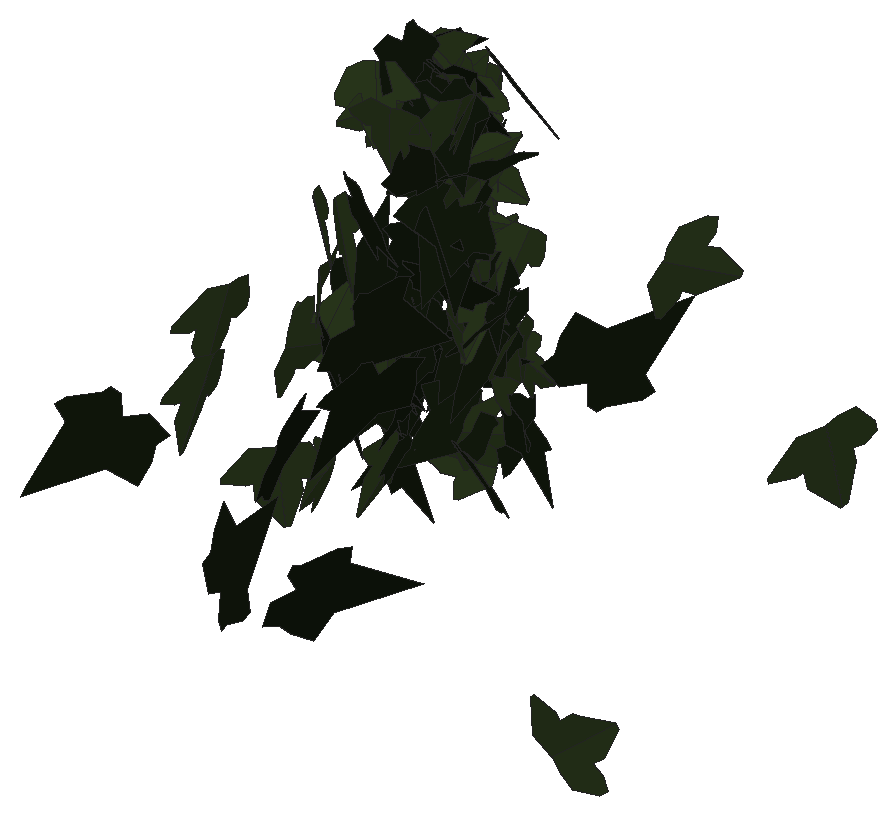
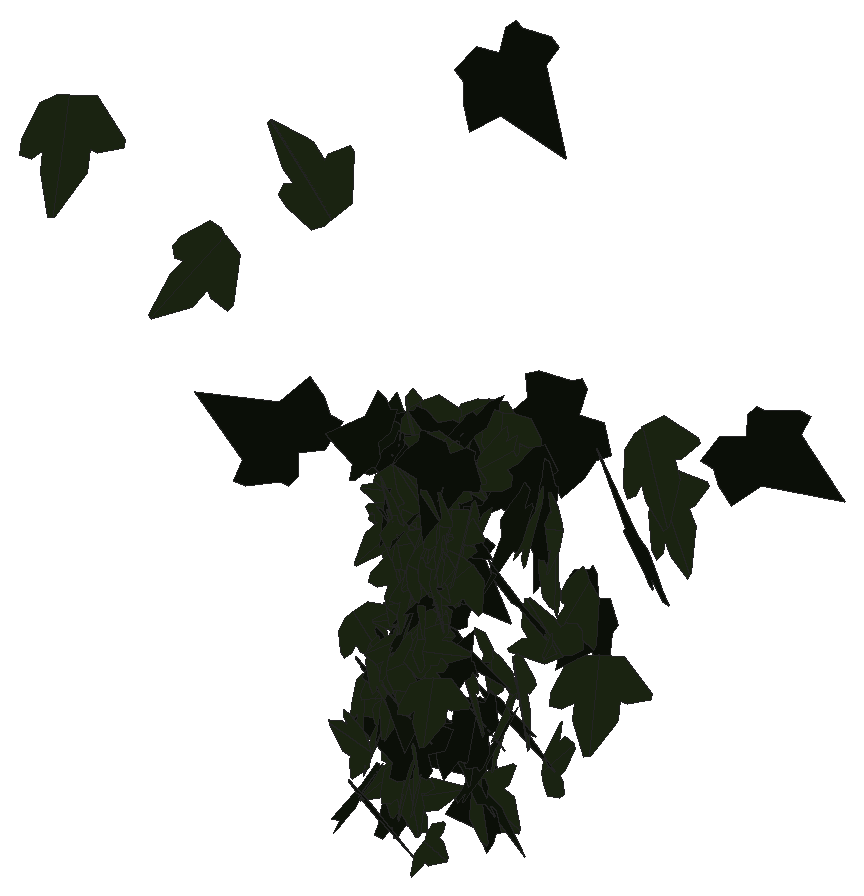
# SketchUp Ruby script. Lengths in inches.
U = 1.inch
M = Sketchup.active_model
def pt(a) = Geom::Point3d.new(a.map { |v| v * U })
def face(e, loops, mat)
  f = e.add_face(loops[0].map { |a| pt(a) })
  loops[1..].each { |l| e.add_face(l.map { |a| pt(a) }).erase! }
  f.material = f.back_material = mat if mat
  f
end
# faces: each face lists its corners as indices into pts; further lists are holes
def faces(e, pts, list, mat = nil) = list.each { |f| face(e, (f[0].is_a?(Array) ? f : [f]).map { |l| l.map { |i| pts[i] } }, mat) }
# xy, xz, yz: faces in a plane at the given z, y or x. An outline is a flat list of corners, or four numbers for a rectangle; further outlines are holes
def ring(l) = l.size == 4 ? [[l[0], l[1]], [l[2], l[1]], [l[2], l[3]], [l[0], l[3]]] : l.each_slice(2).to_a
def flat(e, list, mat, &to3) = list.each { |f| face(e, (f[0].is_a?(Array) ? f : [f]).map { |l| ring(l).map { |u, v| to3.(u, v) } }, mat) }
def xy(e, z, list, mat = nil) = flat(e, list, mat) { |x, y| [x, y, z] }
def xz(e, y, list, mat = nil) = flat(e, list, mat) { |x, z| [x, y, z] }
def yz(e, x, list, mat = nil) = flat(e, list, mat) { |y, z| [x, y, z] }
def lines(e, pts, list) = list.each { |a, b| e.add_line(pt(pts[a]), pt(pts[b])) }
# prism: a flat outline (further loops are holes) pulled along v
def prism(e, loops, v, mat = nil)
  f = face(e, loops, mat); d = Geom::Vector3d.new(v.map { |x| x * U })
  f.pushpull(f.normal.samedirection?(d) ? d.length : -d.length)
end
def box(e, o, s, mat = nil) = prism(e, [[o, [o[0] + s[0], o[1], o[2]], [o[0] + s[0], o[1] + s[1], o[2]], [o[0], o[1] + s[1], o[2]]]], [0, 0, s[2]], mat)
def at(x, y, z, deg = 0) = Geom::Transformation.translation(pt([x, y, z])) * Geom::Transformation.rotation(ORIGIN, Z_AXIS, deg.degrees)
def axes(o, x, y, z) = Geom::Transformation.new([*x, 0, *y, 0, *z, 0, *pt(o).to_a, 1])
def part(name) = M.definitions.add(name)
# library, detail: a bought-in or finely detailed component or shape, given as its bounding box
def library(name, o, s) = part(name).tap { |d| box(d.entities, o, s) }
def detail(e, o, s) = box(e.add_group.entities, o, s)
def put(e, d, t, mat = nil) = e.add_instance(d, t).tap { |i| i.material = mat if mat }
def group(e, t, mat = nil) = e.add_group.tap { |g| g.transformation = t; g.material = mat if mat }.entities
root = M.entities
M.materials.add("efeu1").color = [18, 25, 13]
M.materials.add("efeu2").color = [43, 57, 29]
c1 = part("ivyleaf_10")
p = [[0,0.5,-0.03],[-0.0625,2.02,-0.43],[-0.19,2.01,-0.46],[-0.54,1.05,-0.29],[-0.52,0.625,-0.18],[-0.83,0.76,-0.28],
  [-1.16,0.64,-0.33],[-1.15,0.33,-0.24],[-0.77,-0.39,0.02],[-0.3,-0.51,0.16],[0.04,-0.48,0.23],[-0.02,2.01,-0.4375],
  [-0.06,2.01,-0.43],[0.04,-0.49,0.23],[0.67,-0.49,0.14],[1.38,0.36,-0.2],[1.375,0.51,-0.24],[0.81,0.65,-0.19],
  [0.62,0.59,-0.15],[0.6,1.09,-0.28],[0.5,1.23,-0.31]]
faces(c1.entities,p,[[0,1,2,3,4,5,6,7,8,9,10],[11,12,0,13,14,15,16,17,18,19,20]],"efeu2")
c2 = part("ivyleaf_9")
p = [[1.54,2.16,1.25],[1.36,2.04,1.19],[-0.21,0.99,0.68],[-0.71,1.11,0.82],[-0.85,0.86,0.67],[-0.8,0.17,0.21],
  [-0.9,-0.01,0.1],[-0.67,-0.16,-0.02],[-0.08,-0.08,-0.05],[-0.03,-0.6,-0.4],[0.65,-0.88,-0.66],[0.83,-0.6,-0.49],
  [1.29,-0.42,-0.43],[1.8125,-0.07,-0.26],[1.21,0.44,0.15]]
faces(c2.entities,p,[[0,1,2,3,4,5,6,7,8,9,10,11,12,13,14]],"efeu1")
put(root,c1,axes([618.1,118.79,177.4],[-0.80128,-0.13054,0.8762],[0.86462,0.14198,0.81185],[-0.19287,1.17882,-0.00075]))
put(root,c2,axes([610.8,120.43,184.88],[-0.23488,0.76108,-0.84981],[0.19589,-0.82784,-0.79555],[-1.12385,-0.30336,0.03894]))
put(root,c2,axes([600.09,123.48,178.59],[0.0174,0.18419,-1.07806],[-0.19273,-1.06081,-0.18436],[-1.07657,0.19289,0.01558]))
put(root,c2,axes([606.75,122.49,176.47],[0.00765,0.49498,-1.03911],[0.05876,1.03761,0.4947],[1.14948,-0.05634,-0.01838]))
put(root,c2,axes([602.61,124.54,174.1875],[-0.37072,0.74077,0.89729],[0.40287,-0.80177,0.82835],[1.09159,0.54748,-0.00098]))
put(root,c1,axes([599.92,127.11,178.3],[0.12206,-1.07652,0.27805],[0.0913,-0.26907,-1.08184],[1.1081,0.14076,0.05851]))
put(root,c1,axes([600.05,127.7,180.18],[-0.09973,-1.11378,0.12529],[0.00395,-0.12613,-1.11814],[1.1208,-0.09866,0.01509]))
put(root,c1,axes([619.55,127.58,183.08],[-0.47837,-1.10896,-0.32044],[0.12629,0.29451,-1.20774],[1.1474,-0.49476,-0.00066]))
put(root,c2,axes([601.7,129.82,178.38],[0.16973,0.00062,-1.15833],[1.14995,-0.14064,0.16843],[-0.13907,-1.16222,-0.021]))
put(root,c2,axes([601.04,128.6875,175.7],[-0.26204,0.36444,-0.95279],[-0.69432,0.65698,0.44225],[0.74736,0.73814,0.0768]))
put(root,c1,axes([599.92,130.08,174.46],[-0.72017,-0.76846,-0.08968],[0.08968,0.03878,-1.05246],[0.76846,-0.7247,0.03878]))
put(root,c2,axes([603.09,129.35,179.72],[0.0011,0.12319,-1.16749],[-0.37975,1.10476,0.11621],[1.11085,0.37754,0.04088]))
put(root,c1,axes([599.67,130.97,177.32],[-0.03805,-0.46494,-0.9417],[0.09158,0.93726,-0.46644],[1.04622,-0.09895,0.00658]))
put(root,c1,axes([599.46,132.55,172.98],[0.03898,-0.06049,0.83472],[0.42091,-0.72083,-0.07189],[0.72336,0.4227,-0.00314]))
put(root,c1,axes([599.39,132.59,178.22],[0.16066,-0.52835,-0.63071],[0.18604,-0.60265,0.55223],[-0.80146,-0.2458,0.00175]))
put(root,c1,axes([611.57,131.51,183.64],[-0.23737,-0.55953,-0.98755],[0.43074,0.88903,-0.60725],[1.05014,-0.49114,0.02586]))
put(root,c1,axes([599.18,132.69,180.26],[-0.23627,0.36051,-0.71898],[0.41315,-0.58854,-0.43087],[-0.69007,-0.47579,-0.0118]))
put(root,c2,axes([608.52,131.91,179.03],[-0.10218,-0.07352,1.13697],[1.0678,0.39198,0.12131],[-0.39739,1.07215,0.03361]))
put(root,c1,axes([599.96,132.59,180.38],[-0.34805,0.85303,-0.18752],[0.07171,-0.17326,-0.9213],[-0.87044,-0.35536,-0.00093]))
put(root,c1,axes([599.36,132.48,176.62],[0.69189,0.31446,-0.369],[0.33043,0.16468,0.7599],[0.35477,-0.76665,0.01188]))
put(root,c2,axes([600.01,133.07,180.625],[0.72563,-0.24194,-0.53895],[-0.48083,0.25408,-0.76144],[0.34322,0.86744,0.07271]))
put(root,c1,axes([600.99,133.32,183.24],[-0.86884,-0.19339,0.14525],[-0.14369,-0.02296,-0.89006],[0.19455,-0.8806,-0.00869]))
put(root,c1,axes([599.81,133.44,176.01],[0.41531,-0.80896,-0.29533],[-0.11661,0.27204,-0.90913],[0.85326,0.43093,0.0195]))
put(root,c2,axes([600.27,133.86,175.28],[-0.9117,0.06496,-0.21931],[0.21569,-0.05574,-0.91317],[-0.07612,-0.93604,0.03916]))
put(root,c2,axes([600.04,133.21,177.92],[-0.74342,0.51685,0.11306],[0.08693,-0.07302,0.90538],[0.52189,0.74842,0.01026]))
put(root,c1,axes([600.24,133.89,176.5625],[0.74068,-0.23373,0.42112],[0.40768,-0.10708,-0.77647],[0.25645,0.84527,0.01808]))
put(root,c1,axes([599.89,134.51,182.71],[-0.12686,0.14223,0.83008],[0.06692,-0.83509,0.15331],[0.83951,0.08806,0.11321]))
put(root,c1,axes([599.92,133.93,183.73],[0.78689,0.34669,0.13669],[0.12304,0.05977,-0.85986],[-0.35177,0.79643,0.00502]))
put(root,c1,axes([600.02,134.6,172.74],[0.07965,-0.64529,0.60282],[0.09925,-0.5949,-0.64992],[0.87747,0.12586,0.01879]))
put(root,c1,axes([599.79,133.91,175.28],[-0.44822,0.79806,0.12168],[-0.06404,0.10359,-0.9153],[-0.80474,-0.45274,0.00507]))
put(root,c2,axes([602.01,134.7,180.34],[-0.51357,-0.73059,-0.04307],[0.02436,0.03552,-0.89304],[0.73146,-0.51414,-0.0005]))
put(root,c2,axes([601.41,134.52,179.48],[0.0033,0.35405,-0.78387],[-0.25367,-0.74861,-0.33919],[-0.82186,0.23248,0.10154]))
put(root,c1,axes([602.08,134.53,183.32],[-0.23219,-0.87367,0.10082],[-0.02636,-0.09732,-0.90399],[0.87907,-0.23368,-0.00048]))
put(root,c1,axes([601.58,134.47,182.68],[-0.5117,0.00828,0.71],[-0.68529,-0.23482,-0.49115],[0.18584,-0.84308,0.14377]))
put(root,c2,axes([602.88,135.1,181.89],[-0.35872,-0.81464,0.01399],[0.8047,-0.35663,-0.13333],[0.12761,-0.04108,0.88008]))
put(root,c2,axes([601.72,134.97,179.83],[0.09499,-0.86539,0.18702],[0.00536,-0.18752,-0.87047],[0.88536,0.09399,-0.01479]))
put(root,c2,axes([601.54,134.66,183.43],[-0.39607,-0.46701,-0.61897],[0.48408,0.39403,-0.60704],[0.60571,-0.62027,0.0804]))
put(root,c2,axes([600.5,134.51,173.44],[-0.70031,0.57203,-0.08712],[0.0685,-0.05385,-0.90424],[-0.57456,-0.70365,-0.00163]))
put(root,c2,axes([601.18,134.18,180.98],[-0.0513,-0.1793,0.84576],[0.76318,0.38869,0.1287],[-0.40622,0.7529,0.13498]))
put(root,c2,axes([599.93,134.72,172.74],[-0.02871,-0.03299,-0.75949],[0.73925,0.17603,-0.03559],[0.17728,-0.73937,0.02541]))
put(root,c2,axes([599.75,134.89,174.875],[0.43659,-0.05962,-0.62087],[0.62019,-0.03908,0.43986],[-0.06631,-0.758,0.02616]))
put(root,c1,axes([602.35,134.68,183.48],[0.40574,-0.80316,-0.13013],[-0.07343,0.10868,-0.89968],[0.81032,0.41201,-0.01637]))
put(root,c2,axes([601.34,134.83,177.81],[0.82406,0.15537,0.12513],[-0.13804,0.06015,0.83438],[0.14403,-0.83133,0.08376]))
put(root,c2,axes([600.52,135.23,175.15],[-0.21588,0.33588,-0.72797],[0.38856,-0.61561,-0.39926],[-0.70127,-0.44449,0.00288]))
put(root,c2,axes([600.99,134.85,176.01],[-0.59083,0.48466,0.36369],[-0.28089,0.23102,-0.76418],[-0.5369,-0.6542,-0.00043]))
put(root,c2,axes([600.05,134.97,184.28],[0.28303,-0.61832,-0.45557],[-0.16948,0.42327,-0.67977],[0.74909,0.32938,0.01834]))
put(root,c2,axes([601.77,135.5625,174.1],[-0.70793,-0.31325,0.23577],[-0.19979,-0.13049,-0.77327],[0.33734,-0.73466,0.03682]))
put(root,c2,axes([601.22,135.6875,182.71],[-0.12328,-0.7873,0.23501],[0.00489,-0.23834,-0.79589],[0.82161,-0.11671,0.04]))
put(root,c2,axes([599.77,135.58,173.64],[0.30902,-0.76459,0.02987],[0.01649,0.03885,0.82413],[-0.76499,-0.30802,0.02982]))
put(root,c1,axes([600.28,134.97,176.37],[0.32904,-0.39576,-0.57264],[-0.37546,0.43245,-0.51461],[0.58615,0.49917,-0.00818]))
put(root,c2,axes([600.79,135.74,182.9375],[0.10544,-0.7065,0.26288],[0.05531,-0.25747,-0.71415],[0.75179,0.11803,0.01567]))
put(root,c1,axes([601.95,135.64,172.61],[-0.15419,-0.03304,-0.78548],[-0.75136,-0.2294,0.15714],[-0.23139,0.7669,0.01316]))
put(root,c2,axes([600.61,135.59,180.89],[-0.3809,-0.56241,-0.48282],[0.3526,0.34001,-0.67422],[0.652,-0.51244,0.08255]))
put(root,c1,axes([601.93,134.98,180.51],[0.0872,-0.45049,0.76235],[-0.03505,0.76368,0.45529],[-0.88481,-0.07465,0.05709]))
put(root,c2,axes([600.42,135.41,177.61],[-0.46971,0.32639,0.50895],[-0.41535,0.29414,-0.57197],[-0.43936,-0.627,-0.00339]))
put(root,c2,axes([601.98,135.94,171.96],[0.50057,-0.60501,0.06345],[-0.02155,0.06448,0.78486],[-0.60794,-0.50043,0.02442]))
put(root,c1,axes([601.64,135.12,181.46],[0.17572,0.13816,-0.8179],[0.62405,0.52876,0.22339],[0.54645,-0.64827,0.00789]))
put(root,c1,axes([600.55,135.59,183.02],[-0.61782,-0.48272,-0.06297],[0.05123,0.03671,-0.78403],[0.4841,-0.61993,0.00261]))
put(root,c1,axes([601.45,135.22,176.84],[-0.38162,0.42829,0.59903],[-0.40769,0.43897,-0.57358],[-0.61323,-0.55837,0.00855]))
put(root,c2,axes([601.71,135.38,179.99],[-0.53206,0.64885,0.05088],[0.02233,-0.04748,0.839],[0.65046,0.53237,0.01282]))
put(root,c2,axes([601.8125,136.16,175.97],[-0.71988,-0.08211,-0.33222],[0.33484,-0.00923,-0.72328],[0.07066,-0.79279,0.04282]))
put(root,c2,axes([601.39,136.27,175.82],[-0.74398,-0.2327,-0.09939],[0.09536,0.02806,-0.77953],[0.23438,-0.75007,0.00167]))
put(root,c1,axes([601.875,135.48,173.64],[-0.1469,-0.3112,-0.73197],[0.36078,0.6373,-0.34335],[0.70884,-0.38886,0.02307]))
put(root,c1,axes([600.36,136.4,182.81],[0.02418,-0.23651,-0.6799],[0.44151,-0.53244,0.20091],[-0.56857,-0.42351,0.1271]))
put(root,c2,axes([601.4375,135.79,182.87],[0.74291,0.10167,-0.35465],[-0.35258,-0.03911,-0.74979],[-0.10862,0.82229,0.00819]))
put(root,c1,axes([599.75,135.74,180.64],[-0.25853,0.93196,-0.36339],[-0.11137,0.34618,0.96705],[0.99408,0.28115,0.01383]))
put(root,c2,axes([600.67,135.84,183.38],[0.4845,0.4582,-0.40223],[-0.35419,-0.20667,-0.66206],[-0.49628,0.59483,0.07981]))
put(root,c2,axes([600.34,136.125,176.83],[-0.4834,-0.58149,0.19912],[0.13827,0.14395,0.75606],[-0.59889,0.5026,0.01383]))
put(root,c1,axes([600.23,136.6,180.44],[-0.02911,-0.29855,0.61547],[0.04515,-0.61552,-0.29644],[0.68256,0.02798,0.04586]))
put(root,c1,axes([601.25,136.34,180.68],[0.11401,-0.7578,0.17561],[0.05029,-0.16994,-0.76596],[0.77625,0.12231,0.02383]))
put(root,c1,axes([600.32,136.08,182.65],[-0.69286,-0.05354,0.28431],[-0.28125,-0.0483,-0.69449],[0.06781,-0.74736,0.02452]))
put(root,c2,axes([600.68,136.71,179.17],[-0.13345,-0.72679,0.29694],[-0.04147,-0.29425,-0.73885],[0.78401,-0.13928,0.01146]))
put(root,c1,axes([601.66,136.42,176.62],[0.53338,0.43394,-0.30362],[-0.23097,-0.19718,-0.68757],[-0.47659,0.58121,-0.00658]))
put(root,c2,axes([602.14,136.49,183.51],[0.50007,-0.48001,0.43659],[0.32432,-0.29251,-0.69307],[0.56199,0.59592,0.01148]))
put(root,c1,axes([601.78,135.78,180.96],[0.19218,0.47738,0.64728],[0.22051,0.60873,-0.51442],[-0.77346,0.29216,0.01417]))
put(root,c1,axes([601.38,136.26,173.67],[-0.68625,0.01569,0.35719],[-0.3575,-0.04105,-0.68504],[0.00506,-0.77255,0.04366]))
put(root,c1,axes([601.03,136.52,182.64],[-0.74876,-0.05012,-0.27636],[0.27501,-0.29066,-0.6924],[-0.05705,-0.74333,0.28938]))
put(root,c2,axes([602.42,136.39,176.4],[-0.70383,0.37249,0.21429],[-0.18554,0.10751,-0.79628],[-0.38761,-0.72783,-0.00795]))
put(root,c1,axes([600.18,136.08,183.72],[0.43365,0.38238,0.48901],[0.20978,0.47114,-0.55444],[-0.58423,0.45299,0.16388]))
put(root,c1,axes([601.37,136.63,181.02],[0.5818,-0.24084,0.46021],[0.44509,-0.12506,-0.62813],[0.26776,0.73119,0.04415]))
put(root,c1,axes([600.59,136.43,178.46],[-0.54292,0.2703,-0.30513],[0.27679,-0.12863,-0.60644],[-0.29925,-0.60936,-0.00734]))
put(root,c2,axes([600.56,136.09,183.11],[0.68793,-0.00064,-0.44396],[-0.42909,0.20912,-0.6652],[0.11391,0.79159,0.17537]))
put(root,c2,axes([601.71,135.94,176.24],[-0.01948,0.75894,0.37765],[-0.2275,0.35921,-0.73362],[-0.81661,-0.11818,0.19537]))
put(root,c2,axes([600.55,136.44,174.77],[0.2752,-0.14159,0.70585],[0.69717,-0.13602,-0.2991],[0.17952,0.74529,0.0795]))
put(root,c1,axes([599.87,136.43,181.5],[-0.44958,0.58765,0.02322],[-0.01493,0.01781,-0.7399],[-0.58792,-0.44983,0.00104]))
put(root,c1,axes([599.81,137.07,180.98],[0.01367,-0.42646,0.5977],[0.07088,-0.59424,-0.42562],[0.73081,0.06561,0.0301]))
put(root,c1,axes([600.87,136.58,181.11],[-0.04336,-0.79501,-0.09733],[-0.00176,0.09757,-0.79616],[0.80095,-0.04282,-0.00702]))
put(root,c2,axes([601.42,136.8,177.6875],[-0.42885,-0.16914,-0.62901],[0.62169,0.1184,-0.4557],[0.19433,-0.75203,0.06972]))
put(root,c1,axes([602.44,136.47,175.99],[0.04774,-0.76718,-0.28533],[0.03515,0.28747,-0.76706],[0.81777,0.03243,0.04963]))
put(root,c1,axes([599.91,136.84,181.03],[-0.39314,-0.56195,0.30563],[-0.16725,-0.25597,-0.68576],[0.61744,-0.42714,0.00885]))
put(root,c1,axes([601,136.7,180.27],[0.75736,-0.19991,0.11823],[0.13837,0.0645,-0.77732],[0.18654,0.76381,0.09659]))
put(root,c2,axes([599.94,136.23,183.71],[0.38959,0.68385,-0.04177],[-0.03106,-0.03037,-0.78695],[-0.68442,0.39065,0.01194]))
put(root,c1,axes([602.21,136.1,175.04],[-0.23655,0.32204,0.73224],[-0.40198,0.61231,-0.39915],[-0.69159,-0.46605,-0.01845]))
put(root,c1,axes([599.13,136.71,180.73],[-0.61025,-0.10632,-0.51653],[0.52732,-0.13209,-0.59582],[-0.00605,-0.78852,0.16945]))
put(root,c2,axes([599.73,136.7,180],[0.20854,-0.66223,-0.3633],[-0.00491,0.3757,-0.68764],[0.75532,0.18528,0.09584]))
put(root,c1,axes([601.43,136.6,176.52],[-0.70564,0.24489,0.03144],[-0.03035,0.00844,-0.74692],[-0.24503,-0.70628,0.00198]))
put(root,c1,axes([600.03,137.16,178.7],[-0.04781,0.27412,-0.61443],[-0.14461,-0.60577,-0.259],[-0.65708,0.11338,0.10171]))
put(root,c1,axes([599.55,136.62,181.98],[-0.22673,-0.71632,-0.2254],[0.08498,0.20946,-0.75115],[0.74612,-0.24153,0.01706]))
put(root,c1,axes([600.3125,136.46,178.92],[-0.10924,-0.09476,-0.73448],[0.69105,0.25389,-0.13554],[0.26627,-0.69781,0.05043]))
put(root,c1,axes([600.23,136.8,182],[-0.30405,0.60529,-0.18977],[0.08452,-0.16991,-0.67736],[-0.62868,-0.31558,0.00071]))
put(root,c1,axes([600.33,136.5625,179.1],[0.35078,0.51922,0.37715],[0.2127,0.31146,-0.62661],[-0.60547,0.41023,-0.00162]))
put(root,c1,axes([600.49,136.88,177.71],[0.568,-0.05209,-0.42582],[-0.42349,0.04478,-0.57037],[0.06853,0.70848,0.00474]))
put(root,c2,axes([602.18,137.07,173.21],[0.38521,-0.67238,0.08197],[0.0439,-0.06932,-0.7749],[0.67593,0.38768,0.00361]))
put(root,c1,axes([600.17,136.45,181.39],[-0.05246,0.06508,-0.70544],[-0.42142,0.56573,0.08353],[0.56945,0.42467,-0.00317]))
put(root,c1,axes([602.12,137.2,178.43],[-0.29325,-0.56059,0.37592],[0.0375,-0.42277,-0.6012],[0.67392,-0.22041,0.19704]))
put(root,c1,axes([600.03,137.21,178.38],[0.18549,0.1526,-0.62744],[-0.45381,-0.43361,-0.23962],[-0.45938,0.48997,-0.01664]))
put(root,c1,axes([600.87,136.6875,174.29],[-0.42032,0.56779,0.11249],[-0.08141,0.07964,-0.70621],[-0.57307,-0.42776,0.01783]))
put(root,c1,axes([601.66,137.07,177.51],[0.18479,-0.73184,0.13191],[0.03818,-0.12641,-0.75478],[0.74265,0.1886,0.00598]))
put(root,c1,axes([600.76,136.89,180.3125],[-0.73384,-0.26816,-0.13173],[0.14394,-0.01121,-0.77906],[0.2618,-0.74548,0.0591]))
put(root,c2,axes([602.25,136.94,173.07],[-0.6645,0.36511,0.18835],[-0.15715,0.10503,-0.75803],[-0.37958,-0.68265,-0.01589]))
put(root,c1,axes([600.7,136.57,174],[0.10188,-0.11012,0.73702],[-0.54718,0.49393,0.14944],[-0.50588,-0.55643,-0.0132]))
put(root,c1,axes([600.09,136.93,182.54],[-0.71965,0.08511,0.17442],[-0.17654,-0.00885,-0.7241],[-0.08062,-0.74044,0.0287]))
put(root,c1,axes([600.08,137.06,182.32],[0.55991,-0.13537,-0.48508],[0.46473,-0.14057,0.57566],[-0.19402,-0.72735,-0.02098]))
put(root,c1,axes([600.73,137.26,181.19],[0.23558,0.16747,0.66778],[-0.5278,-0.40925,0.28883],[0.44205,-0.57788,-0.01102]))
put(root,c1,axes([600.3,136.81,180.17],[-0.2328,0.57275,0.37531],[-0.36576,0.23111,-0.57957],[-0.57889,-0.37636,0.21526]))
put(root,c1,axes([600.48,137.62,177.84],[-0.01253,0.02833,0.67814],[0.07424,-0.67413,0.02954],[0.67466,0.07471,0.00935]))
put(root,c1,axes([600.66,136.86,179.98],[-0.15649,0.66075,0.24701],[-0.1718,0.2097,-0.66978],[-0.68417,-0.20378,0.11169]))
put(root,c1,axes([601.11,137.26,182.59],[0.5515,-0.43188,0.01125],[0.00868,-0.00716,-0.70048],[0.43194,0.55157,-0.00028]))
put(root,c1,axes([599.9,137.63,181],[0.06045,-0.39403,0.56988],[0.24458,-0.52308,-0.38761],[0.64823,0.2341,0.0931]))
put(root,c1,axes([601.92,137.4375,174.93],[-0.05772,0.01632,-0.74835],[0.62405,-0.41342,-0.05714],[-0.41334,-0.62645,0.01822]))
put(root,c1,axes([599.71,137.23,177.19],[-0.45429,-0.59704,-0.08792],[0.15372,-0.00807,-0.73951],[0.58358,-0.46265,0.12635]))
put(root,c1,axes([599.62,137.5,172.84],[0.05163,0.47306,-0.43575],[-0.0908,-0.42741,-0.47477],[-0.63672,0.09931,0.03237]))
put(root,c2,axes([600.76,137.37,178.46],[0.14854,-0.67532,0.32709],[-0.02932,0.32796,0.69043],[-0.74979,-0.14661,0.0378]))
put(root,c1,axes([599.35,137.5,180.39],[0.4364,-0.51554,0.32677],[0.25166,-0.214,-0.6737],[0.55608,0.50143,0.04844]))
put(root,c1,axes([599.71,136.77,181.35],[0.23822,0.38494,0.58832],[0.08282,0.60148,-0.42709],[-0.69817,0.20269,0.15007]))
put(root,c1,axes([601.24,136.67,177.96],[0.18039,0.15461,-0.73651],[0.09798,0.74611,0.18062],[0.74616,-0.13535,0.15434]))
